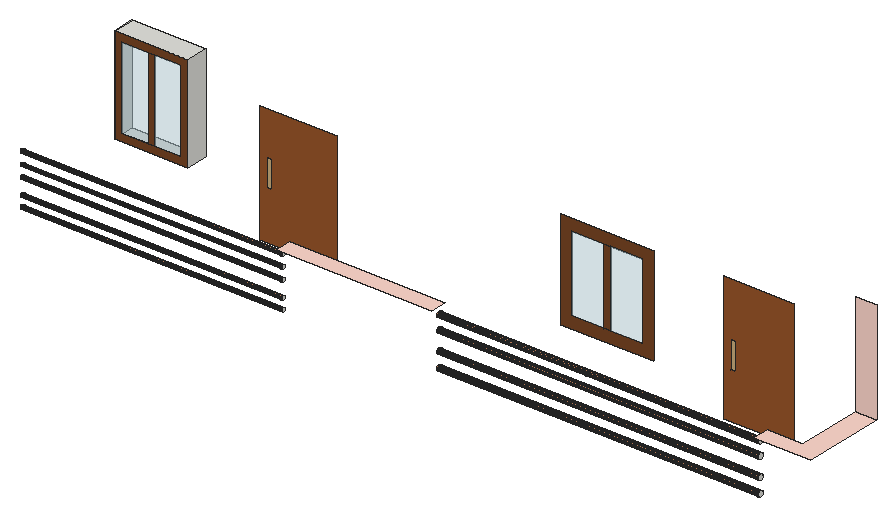
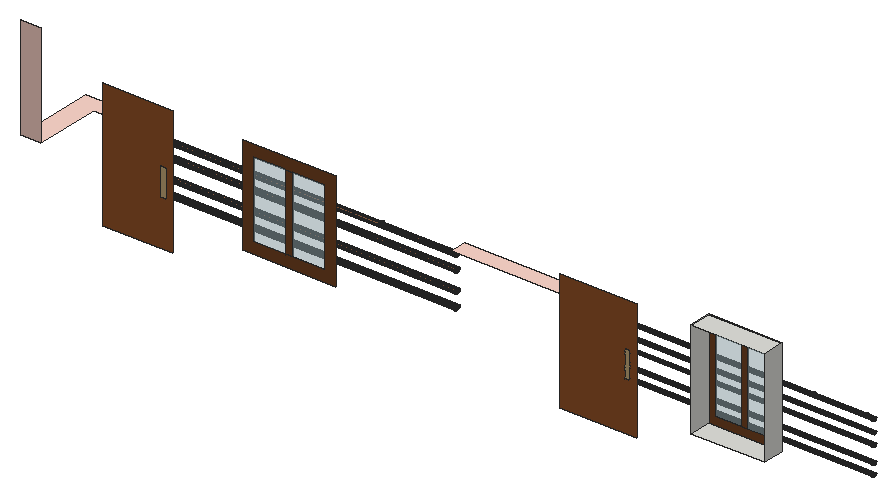
# SketchUp Ruby script. Lengths in inches.
U = 1.inch
M = Sketchup.active_model
def pt(a) = Geom::Point3d.new(a.map { |v| v * U })
def face(e, loops, mat)
  f = e.add_face(loops[0].map { |a| pt(a) })
  loops[1..].each { |l| e.add_face(l.map { |a| pt(a) }).erase! }
  f.material = f.back_material = mat if mat
  f
end
# faces: each face lists its corners as indices into pts; further lists are holes
def faces(e, pts, list, mat = nil) = list.each { |f| face(e, (f[0].is_a?(Array) ? f : [f]).map { |l| l.map { |i| pts[i] } }, mat) }
# xy, xz, yz: faces in a plane at the given z, y or x. An outline is a flat list of corners, or four numbers for a rectangle; further outlines are holes
def ring(l) = l.size == 4 ? [[l[0], l[1]], [l[2], l[1]], [l[2], l[3]], [l[0], l[3]]] : l.each_slice(2).to_a
def flat(e, list, mat, &to3) = list.each { |f| face(e, (f[0].is_a?(Array) ? f : [f]).map { |l| ring(l).map { |u, v| to3.(u, v) } }, mat) }
def xy(e, z, list, mat = nil) = flat(e, list, mat) { |x, y| [x, y, z] }
def xz(e, y, list, mat = nil) = flat(e, list, mat) { |x, z| [x, y, z] }
def yz(e, x, list, mat = nil) = flat(e, list, mat) { |y, z| [x, y, z] }
def lines(e, pts, list) = list.each { |a, b| e.add_line(pt(pts[a]), pt(pts[b])) }
# prism: a flat outline (further loops are holes) pulled along v
def prism(e, loops, v, mat = nil)
  f = face(e, loops, mat); d = Geom::Vector3d.new(v.map { |x| x * U })
  f.pushpull(f.normal.samedirection?(d) ? d.length : -d.length)
end
def box(e, o, s, mat = nil) = prism(e, [[o, [o[0] + s[0], o[1], o[2]], [o[0] + s[0], o[1] + s[1], o[2]], [o[0], o[1] + s[1], o[2]]]], [0, 0, s[2]], mat)
def at(x, y, z, deg = 0) = Geom::Transformation.translation(pt([x, y, z])) * Geom::Transformation.rotation(ORIGIN, Z_AXIS, deg.degrees)
def axes(o, x, y, z) = Geom::Transformation.new([*x, 0, *y, 0, *z, 0, *pt(o).to_a, 1])
def part(name) = M.definitions.add(name)
# library, detail: a bought-in or finely detailed component or shape, given as its bounding box
def library(name, o, s) = part(name).tap { |d| box(d.entities, o, s) }
def detail(e, o, s) = box(e.add_group.entities, o, s)
def put(e, d, t, mat = nil) = e.add_instance(d, t).tap { |i| i.material = mat if mat }
def group(e, t, mat = nil) = e.add_group.tap { |g| g.transformation = t; g.material = mat if mat }.entities
root = M.entities
M.materials.add("[Color B01]").color = [255, 216, 204]
M.materials.add("[Translucent Glass Safety]").color = [204, 235, 244]
M.materials["[Translucent Glass Safety]"].alpha = 0.5
M.materials.add("[Wood Cherry Original]").color = [152, 86, 42]
M.materials.add("[Wood Floor Light]").color = [204, 176, 127]
M.materials.add("[Wood Veneer 01]1").color = [120, 70, 37]
M.materials.add("[Wood Veneer 02]").color = [190, 128, 91]
xy(root,2135.23,[[206.78,571.9,480.91,653.97]])
xy(root,2168.9375,[[2479.625,285.86,2482.375,286.22,2484.9375,287.28,2487.14,288.97,2488.83,291.17,2489.89,293.73,2490.25,296.48,2489.89,299.23,2488.83,301.79,2487.14,303.99,2484.9375,305.68,2482.375,306.74,2479.625,307.11,2476.875,306.74,2474.3125,305.68,2472.11,303.99,2470.42,301.79,2469.36,299.23,2469,296.48,2469.36,293.73,2470.42,291.17,2472.11,288.97,2474.3125,287.28,2476.875,286.22]],"[Wood Veneer 02]")
xy(root,2169.25,[[530.58,291.11,532.59,291.37,534.45,292.15,536.06,293.38,537.29,294.98,538.07,296.85,538.33,298.86,538.07,300.86,537.29,302.73,536.06,304.34,534.45,305.57,532.59,306.34,530.58,306.61,528.57,306.34,526.7,305.57,525.1,304.34,523.87,302.73,523.09,300.86,522.83,298.86,523.09,296.85,523.87,294.98,525.1,293.38,526.7,292.15,528.57,291.37]])
xy(root,2169.6875,[[2192.5,285.86,2195.25,286.22,2197.8125,287.28,2200.01,288.97,2201.7,291.17,2202.76,293.73,2203.125,296.48,2202.76,299.23,2201.7,301.79,2200.01,303.99,2197.8125,305.68,2195.25,306.74,2192.5,307.11,2189.75,306.74,2187.1875,305.68,2184.99,303.99,2183.3,301.79,2182.24,299.23,2181.875,296.48,2182.24,293.73,2183.3,291.17,2184.99,288.97,2187.1875,287.28,2189.75,286.22]],"[Wood Veneer 02]")
xy(root,2170.12,[[988.02,291.11,990.02,291.37,991.89,292.15,993.5,293.38,994.73,294.98,994.75,295.02,981.29,295.02,981.31,294.98,982.54,293.38,984.14,292.15,986.01,291.37],[981.29,295.02,994.75,295.02,995.5,296.85,995.77,298.86,995.5,300.86,994.73,302.73,993.5,304.34,991.89,305.57,990.02,306.34,988.02,306.61,986.01,306.34,984.14,305.57,982.54,304.34,981.31,302.73,980.53,300.86,980.27,298.86,980.53,296.85]])
xy(root,2170.6875,[[748.77,291.11,750.77,291.37,752.64,292.15,754.25,293.38,755.48,294.98,756.25,296.85,756.52,298.86,756.25,300.86,755.48,302.73,754.25,304.34,752.64,305.57,750.77,306.34,748.77,306.61,746.76,306.34,744.89,305.57,743.29,304.34,742.06,302.73,741.28,300.86,741.02,298.86,741.28,296.85,742.06,294.98,743.29,293.38,744.89,292.15,746.76,291.37]])
xy(root,2171.4375,[[1711.75,285.86,1714.5,286.22,1717.0625,287.28,1719.26,288.97,1720.95,291.17,1722.01,293.73,1722.375,296.48,1722.01,299.23,1720.95,301.79,1719.26,303.99,1717.0625,305.68,1714.5,306.74,1711.75,307.11,1709,306.74,1706.4375,305.68,1704.24,303.99,1702.55,301.79,1701.49,299.23,1701.125,296.48,1701.49,293.73,1702.55,291.17,1704.24,288.97,1706.4375,287.28,1709,286.22]])
xy(root,2172.125,[[114.33,291.11,116.34,291.37,118.2,292.15,119.81,293.38,121.04,294.98,121.82,296.85,122.08,298.86,121.82,300.86,121.04,302.73,119.81,304.34,118.2,305.57,116.34,306.34,114.33,306.61,112.32,306.34,110.45,305.57,108.85,304.34,107.62,302.73,106.84,300.86,106.58,298.86,106.84,296.85,107.62,294.98,108.85,293.38,110.45,292.15,112.32,291.37]])
xy(root,2173.03,[[309.08,291.11,311.09,291.37,312.95,292.15,314.56,293.38,315.79,294.98,316.13,295.8,302.03,295.8,302.37,294.98,303.6,293.38,305.2,292.15,307.07,291.37],[302.03,295.8,316.13,295.8,316.57,296.85,316.83,298.86,316.57,300.86,315.79,302.73,314.56,304.34,312.95,305.57,312.23,305.87,305.93,305.87,305.2,305.57,303.6,304.34,302.37,302.73,301.59,300.86,301.33,298.86,301.59,296.85],[305.93,305.87,312.23,305.87,311.09,306.34,309.08,306.61,307.07,306.34]])
xy(root,2173.25,[[2741.25,285.86,2744,286.22,2746.5625,287.28,2748.76,288.97,2750.45,291.17,2751.51,293.73,2751.875,296.48,2751.51,299.23,2750.45,301.79,2748.76,303.99,2746.5625,305.68,2744,306.74,2741.25,307.11,2738.5,306.74,2735.9375,305.68,2733.74,303.99,2732.05,301.79,2730.99,299.23,2730.625,296.48,2730.99,293.73,2732.05,291.17,2733.74,288.97,2735.9375,287.28,2738.5,286.22]],"[Wood Veneer 02]")
xy(root,2176.5,[[1911.67,291.33,1930.2,291.33,1931.2,293.73,1931.5625,296.48,1931.2,299.23,1930.14,301.79,1928.45,303.99,1926.25,305.68,1923.6875,306.74,1921.5625,307.02,1920.3125,307.02,1918.1875,306.74,1915.625,305.68,1913.42,303.99,1911.74,301.79,1910.67,299.23,1910.3125,296.48,1910.67,293.73],[1920.3125,307.02,1921.5625,307.02,1920.9375,307.11]])
xy(root,2176.5,[[1920.9375,285.86,1923.6875,286.22,1926.25,287.28,1928.45,288.97,1930.14,291.17,1930.2,291.33,1911.67,291.33,1911.74,291.17,1913.42,288.97,1915.625,287.28,1918.1875,286.22]],"[Wood Veneer 02]")
xy(root,2195.8125,[[1053.15,267.5625,1631.4,328.8],[2829.41,267.5625,3040.15,267.5625,3040.15,571.9,2962.22,571.9,2962.22,328.8,2829.41,328.8]],"[Color B01]")
xy(root,2496.04,[[206.78,571.9,480.91,653.97]])
xz(root,571.9,[[2962.22,2195.8125,3040.15,2577.9375]],"[Color B01]")
xz(root,571.9,[[1909.23,2143.05,2027.6,2427.3],[2054.17,2143.05,2170.86,2427.3],[235.06,2163.5,333.67,2467.76],[357.21,2163.5,452.63,2467.76]],"[Translucent Glass Safety]")
xz(root,571.9,[[[747.7,1990.6,1033.12,2436.59],[772.37,2170.62,791.56,2274.62]],[[2473.97,2001.07,2732.77,2474.99],[2500.06,2170.62,2519.25,2274.62]]],"[Wood Cherry Original]")
xz(root,571.9,[[772.37,2170.62,791.56,2274.62],[2500.06,2170.62,2519.25,2274.62]],"[Wood Floor Light]")
xz(root,571.9,[[[1867.29,2101.11,2212.79,2469.24],[1909.23,2143.05,2170.86,2427.3]],[[206.78,2135.23,480.91,2496.04],[235.06,2163.5,452.63,2467.76]],[2027.6,2143.05,2054.17,2427.3],[333.67,2163.5,357.21,2467.76]],"[Wood Veneer 01]1")
yz(root,206.78,[[571.9,2135.23,653.97,2496.04]])
yz(root,480.91,[[571.9,2135.23,653.97,2496.04]])
yz(root,1053.15,[[300.84,1977.93,302.34,1978.13,303.74,1978.71,304.95,1979.63,305.87,1980.84,306.45,1982.24,306.65,1983.74,306.45,1985.25,305.87,1986.65,304.95,1987.85,303.74,1988.78,302.34,1989.36,300.84,1989.56,299.33,1989.36,297.93,1988.78,296.73,1987.85,295.8,1986.65,295.22,1985.25,295.02,1983.74,295.22,1982.24,295.8,1980.84,296.73,1979.63,297.93,1978.71,299.33,1978.13],[300.84,2017.49,302.34,2017.69,303.74,2018.27,304.95,2019.2,305.87,2020.4,306.45,2021.8,306.65,2023.31,306.45,2024.8125,305.87,2026.21,304.95,2027.42,303.74,2028.34,302.34,2028.92,300.84,2029.12,299.33,2028.92,297.93,2028.34,296.73,2027.42,295.8,2026.21,295.22,2024.8125,295.02,2023.31,295.22,2021.8,295.8,2020.4,296.73,2019.2,297.93,2018.27,299.33,2017.69],[300.84,2076.99,302.34,2077.19,303.74,2077.77,304.95,2078.7,305.87,2079.9,306.45,2081.3,306.65,2082.81,306.45,2084.3125,305.87,2085.71,304.95,2086.92,303.74,2087.84,302.34,2088.42,300.84,2088.62,299.33,2088.42,297.93,2087.84,296.73,2086.92,295.8,2085.71,295.22,2084.3125,295.02,2082.81,295.22,2081.3,295.8,2079.9,296.73,2078.7,297.93,2077.77,299.33,2077.19],[300.84,2119.12,302.34,2119.32,303.74,2119.9,304.95,2120.82,305.87,2122.03,306.45,2123.43,306.65,2124.93,306.45,2126.4375,305.87,2127.84,304.95,2129.04,303.74,2129.97,302.34,2130.55,300.84,2130.74,299.33,2130.55,297.93,2129.97,296.73,2129.04,295.8,2127.84,295.22,2126.4375,295.02,2124.93,295.22,2123.43,295.8,2122.03,296.73,2120.82,297.93,2119.9,299.33,2119.32],[300.84,2164.31,302.34,2164.51,303.74,2165.09,304.95,2166.01,305.87,2167.21,306.45,2168.62,306.65,2170.12,306.45,2171.625,305.87,2173.03,304.95,2174.23,303.74,2175.15,302.34,2175.73,300.84,2175.93,299.33,2175.73,297.93,2175.15,296.73,2174.23,295.8,2173.03,295.22,2171.625,295.02,2170.12,295.22,2168.62,295.8,2167.21,296.73,2166.01,297.93,2165.09,299.33,2164.51]])
yz(root,2829.41,[[299.17,1985.65,301.52,1985.96,303.71,1986.87,305.58,1988.31,307.02,1990.18,307.93,1992.37,308.24,1994.72,307.93,1997.0625,307.02,1999.25,305.58,2001.125,303.71,2002.5625,301.52,2003.47,299.17,2003.78,296.83,2003.47,294.64,2002.5625,292.77,2001.125,291.33,1999.25,290.42,1997.0625,290.11,1994.72,290.42,1992.37,291.33,1990.18,292.77,1988.31,294.64,1986.87,296.83,1985.96],[299.17,2040.72,301.52,2041.02,303.71,2041.93,305.58,2043.37,307.02,2045.25,307.93,2047.43,308.24,2049.78,307.93,2052.125,307.02,2054.31,305.58,2056.1875,303.71,2057.625,301.52,2058.53,299.17,2058.84,296.83,2058.53,294.64,2057.625,292.77,2056.1875,291.33,2054.31,290.42,2052.125,290.11,2049.78,290.42,2047.43,291.33,2045.25,292.77,2043.37,294.64,2041.93,296.83,2041.02],[299.17,2111.15,301.52,2111.46,303.71,2112.37,305.58,2113.81,307.02,2115.68,307.93,2117.87,308.24,2120.22,307.93,2122.5625,307.02,2124.75,305.58,2126.625,303.71,2128.0625,301.52,2128.97,299.17,2129.28,296.83,2128.97,294.64,2128.0625,292.77,2126.625,291.33,2124.75,290.42,2122.5625,290.11,2120.22,290.42,2117.87,291.33,2115.68,292.77,2113.81,294.64,2112.37,296.83,2111.46],[299.17,2162.9,301.52,2163.21,303.71,2164.12,305.58,2165.56,307.02,2167.43,307.93,2169.62,308.24,2171.97,307.93,2174.3125,307.02,2176.5,305.58,2178.375,303.71,2179.8125,301.52,2180.72,299.17,2181.03,296.83,2180.72,294.64,2179.8125,292.77,2178.375,291.33,2176.5,290.42,2174.3125,290.11,2171.97,290.42,2169.62,291.33,2167.43,292.77,2165.56,294.64,2164.12,296.83,2163.21]])
p = [[1053.15,300.84,1977.93],[1053.15,299.33,1978.13],[77.93,299.33,1978.13],[77.93,300.84,1977.93],[1053.15,302.34,1978.13],[77.93,302.34,1978.13],
  [1053.15,297.93,1978.71],[77.93,297.93,1978.71],[1053.15,303.74,1978.71],[77.93,303.74,1978.71],[1053.15,296.73,1979.63],[77.93,296.73,1979.63],
  [1053.15,304.95,1979.63],[77.93,304.95,1979.63],[1053.15,295.8,1980.84],[77.93,295.8,1980.84],[1053.15,305.87,1980.84],[77.93,305.87,1980.84],
  [1053.15,295.22,1982.24],[77.93,295.22,1982.24],[1053.15,306.45,1982.24],[77.93,306.45,1982.24],[1053.15,295.02,1983.74],[77.93,295.02,1983.74],
  [1053.15,306.65,1983.74],[77.93,306.65,1983.74],[1053.15,295.22,1985.25],[77.93,295.22,1985.25],[1053.15,306.45,1985.25],[77.93,306.45,1985.25],
  [1053.15,295.8,1986.65],[77.93,295.8,1986.65],[1053.15,305.87,1986.65],[77.93,305.87,1986.65],[2829.41,299.17,1985.65],[2829.41,296.83,1985.96],
  [1631.4,296.83,1985.96],[1631.4,299.17,1985.65],[2829.41,301.52,1985.96],[1631.4,301.52,1985.96],[2829.41,294.64,1986.87],[1631.4,294.64,1986.87],
  [2829.41,303.71,1986.87],[1631.4,303.71,1986.87],[1053.15,296.73,1987.85],[77.93,296.73,1987.85],[1053.15,304.95,1987.85],[77.93,304.95,1987.85],
  [2829.41,292.77,1988.31],[1631.4,292.77,1988.31],[2829.41,305.58,1988.31],[1631.4,305.58,1988.31],[1053.15,297.93,1988.78],[77.93,297.93,1988.78],
  [1053.15,303.74,1988.78],[77.93,303.74,1988.78],[2829.41,291.33,1990.18],[1631.4,291.33,1990.18],[2829.41,307.02,1990.18],[1631.4,307.02,1990.18],
  [1053.15,299.33,1989.36],[77.93,299.33,1989.36],[1053.15,302.34,1989.36],[77.93,302.34,1989.36],[1053.15,300.84,1989.56],[77.93,300.84,1989.56],
  [2829.41,290.42,1992.37],[1631.4,290.42,1992.37],[2829.41,307.93,1992.37],[1631.4,307.93,1992.37],[2829.41,290.11,1994.72],[1631.4,290.11,1994.72],
  [2829.41,308.24,1994.72],[1631.4,308.24,1994.72],[2829.41,290.42,1997.0625],[1631.4,290.42,1997.0625],[2829.41,307.93,1997.0625],[1631.4,307.93,1997.0625],
  [2829.41,291.33,1999.25],[1631.4,291.33,1999.25],[2829.41,307.02,1999.25],[1631.4,307.02,1999.25],[2829.41,292.77,2001.125],[1631.4,292.77,2001.125],
  [2829.41,305.58,2001.125],[1631.4,305.58,2001.125],[2829.41,294.64,2002.5625],[1631.4,294.64,2002.5625],[2829.41,303.71,2002.5625],[1631.4,303.71,2002.5625],
  [2829.41,296.83,2003.47],[1631.4,296.83,2003.47],[2829.41,301.52,2003.47],[1631.4,301.52,2003.47],[2829.41,299.17,2003.78],[1631.4,299.17,2003.78],
  [1053.15,300.84,2017.49],[1053.15,299.33,2017.69],[77.93,299.33,2017.69],[77.93,300.84,2017.49],[1053.15,302.34,2017.69],[77.93,302.34,2017.69],
  [1053.15,297.93,2018.27],[77.93,297.93,2018.27],[1053.15,303.74,2018.27],[77.93,303.74,2018.27],[1053.15,296.73,2019.2],[77.93,296.73,2019.2],
  [1053.15,304.95,2019.2],[77.93,304.95,2019.2],[1053.15,295.8,2020.4],[77.93,295.8,2020.4],[1053.15,305.87,2020.4],[77.93,305.87,2020.4],
  [1053.15,295.22,2021.8],[77.93,295.22,2021.8],[1053.15,306.45,2021.8],[77.93,306.45,2021.8],[1053.15,295.02,2023.31],[77.93,295.02,2023.31],
  [1053.15,306.65,2023.31],[77.93,306.65,2023.31],[1053.15,295.22,2024.8125],[77.93,295.22,2024.8125],[1053.15,306.45,2024.8125],[77.93,306.45,2024.8125],
  [1053.15,295.8,2026.21],[77.93,295.8,2026.21],[1053.15,305.87,2026.21],[77.93,305.87,2026.21],[1053.15,296.73,2027.42],[77.93,296.73,2027.42],
  [1053.15,304.95,2027.42],[77.93,304.95,2027.42],[1053.15,297.93,2028.34],[77.93,297.93,2028.34],[1053.15,303.74,2028.34],[77.93,303.74,2028.34],
  [1053.15,299.33,2028.92],[77.93,299.33,2028.92],[1053.15,302.34,2028.92],[77.93,302.34,2028.92],[1053.15,300.84,2029.12],[77.93,300.84,2029.12],
  [2829.41,299.17,2040.72],[2829.41,296.83,2041.02],[1631.4,296.83,2041.02],[1631.4,299.17,2040.72],[2829.41,301.52,2041.02],[1631.4,301.52,2041.02],
  [2829.41,294.64,2041.93],[1631.4,294.64,2041.93],[2829.41,303.71,2041.93],[1631.4,303.71,2041.93],[2829.41,292.77,2043.37],[1631.4,292.77,2043.37],
  [2829.41,305.58,2043.37],[1631.4,305.58,2043.37],[2829.41,291.33,2045.25],[1631.4,291.33,2045.25],[2829.41,307.02,2045.25],[1631.4,307.02,2045.25],
  [2829.41,290.42,2047.43],[1631.4,290.42,2047.43],[2829.41,307.93,2047.43],[1631.4,307.93,2047.43],[2829.41,290.11,2049.78],[1631.4,290.11,2049.78],
  [2829.41,308.24,2049.78],[1631.4,308.24,2049.78],[2829.41,290.42,2052.125],[1631.4,290.42,2052.125],[2829.41,307.93,2052.125],[1631.4,307.93,2052.125],
  [2829.41,291.33,2054.31],[1631.4,291.33,2054.31],[2829.41,307.02,2054.31],[1631.4,307.02,2054.31],[2829.41,292.77,2056.1875],[1631.4,292.77,2056.1875],
  [2829.41,305.58,2056.1875],[1631.4,305.58,2056.1875],[2829.41,294.64,2057.625],[1631.4,294.64,2057.625],[2829.41,303.71,2057.625],[1631.4,303.71,2057.625],
  [2829.41,296.83,2058.53],[1631.4,296.83,2058.53],[2829.41,301.52,2058.53],[1631.4,301.52,2058.53],[2829.41,299.17,2058.84],[1631.4,299.17,2058.84],
  [1053.15,300.84,2076.99],[1053.15,299.33,2077.19],[77.93,299.33,2077.19],[77.93,300.84,2076.99],[1053.15,302.34,2077.19],[77.93,302.34,2077.19],
  [1053.15,297.93,2077.77],[77.93,297.93,2077.77],[1053.15,303.74,2077.77],[77.93,303.74,2077.77],[1053.15,296.73,2078.7],[77.93,296.73,2078.7],
  [1053.15,304.95,2078.7],[77.93,304.95,2078.7],[1053.15,295.8,2079.9],[77.93,295.8,2079.9],[1053.15,305.87,2079.9],[77.93,305.87,2079.9],
  [1053.15,295.22,2081.3],[77.93,295.22,2081.3],[1053.15,306.45,2081.3],[77.93,306.45,2081.3],[1053.15,295.02,2082.81],[77.93,295.02,2082.81],
  [1053.15,306.65,2082.81],[77.93,306.65,2082.81],[1053.15,295.22,2084.3125],[77.93,295.22,2084.3125],[1053.15,306.45,2084.3125],[77.93,306.45,2084.3125],
  [1053.15,295.8,2085.71],[77.93,295.8,2085.71],[1053.15,305.87,2085.71],[77.93,305.87,2085.71],[1053.15,296.73,2086.92],[77.93,296.73,2086.92],
  [1053.15,304.95,2086.92],[77.93,304.95,2086.92],[1053.15,297.93,2087.84],[77.93,297.93,2087.84],[1053.15,303.74,2087.84],[77.93,303.74,2087.84],
  [1053.15,299.33,2088.42],[77.93,299.33,2088.42],[1053.15,302.34,2088.42],[77.93,302.34,2088.42],[1053.15,300.84,2088.62],[77.93,300.84,2088.62],
  [2829.41,299.17,2111.15],[2829.41,296.83,2111.46],[1631.4,296.83,2111.46],[1631.4,299.17,2111.15],[2829.41,301.52,2111.46],[1631.4,301.52,2111.46],
  [2829.41,294.64,2112.37],[1631.4,294.64,2112.37],[2829.41,303.71,2112.37],[1631.4,303.71,2112.37],[2829.41,292.77,2113.81],[1631.4,292.77,2113.81],
  [2829.41,305.58,2113.81],[1631.4,305.58,2113.81],[2829.41,291.33,2115.68],[1631.4,291.33,2115.68],[2829.41,307.02,2115.68],[1631.4,307.02,2115.68],
  [2829.41,290.42,2117.87],[1631.4,290.42,2117.87],[2829.41,307.93,2117.87],[1631.4,307.93,2117.87],[2829.41,290.11,2120.22],[1631.4,290.11,2120.22],
  [2829.41,308.24,2120.22],[1631.4,308.24,2120.22],[1053.15,300.84,2119.12],[1053.15,299.33,2119.32],[77.93,299.33,2119.32],[77.93,300.84,2119.12],
  [1053.15,302.34,2119.32],[77.93,302.34,2119.32],[1053.15,297.93,2119.9],[77.93,297.93,2119.9],[1053.15,303.74,2119.9],[77.93,303.74,2119.9],
  [1053.15,296.73,2120.82],[77.93,296.73,2120.82],[1053.15,304.95,2120.82],[77.93,304.95,2120.82],[2829.41,290.42,2122.5625],[1631.4,290.42,2122.5625],
  [2829.41,307.93,2122.5625],[1631.4,307.93,2122.5625],[1053.15,295.8,2122.03],[77.93,295.8,2122.03],[1053.15,305.87,2122.03],[77.93,305.87,2122.03],
  [1053.15,295.22,2123.43],[77.93,295.22,2123.43],[1053.15,306.45,2123.43],[77.93,306.45,2123.43],[2829.41,291.33,2124.75],[1631.4,291.33,2124.75],
  [2829.41,307.02,2124.75],[1631.4,307.02,2124.75],[1053.15,295.02,2124.93],[77.93,295.02,2124.93],[1053.15,306.65,2124.93],[77.93,306.65,2124.93],
  [2829.41,292.77,2126.625],[1631.4,292.77,2126.625],[2829.41,305.58,2126.625],[1631.4,305.58,2126.625],[1053.15,295.22,2126.4375],[77.93,295.22,2126.4375],
  [1053.15,306.45,2126.4375],[77.93,306.45,2126.4375],[1053.15,295.8,2127.84],[77.93,295.8,2127.84],[1053.15,305.87,2127.84],[77.93,305.87,2127.84],
  [2829.41,294.64,2128.0625],[1631.4,294.64,2128.0625],[2829.41,303.71,2128.0625],[1631.4,303.71,2128.0625],[1053.15,296.73,2129.04],[77.93,296.73,2129.04],
  [1053.15,304.95,2129.04],[77.93,304.95,2129.04],[2829.41,296.83,2128.97],[1631.4,296.83,2128.97],[2829.41,301.52,2128.97],[1631.4,301.52,2128.97],
  [1053.15,297.93,2129.97],[77.93,297.93,2129.97],[2829.41,299.17,2129.28],[1631.4,299.17,2129.28],[1053.15,303.74,2129.97],[77.93,303.74,2129.97],
  [1053.15,299.33,2130.55],[77.93,299.33,2130.55],[1053.15,302.34,2130.55],[77.93,302.34,2130.55],[1053.15,300.84,2130.74],[77.93,300.84,2130.74],
  [2829.41,299.17,2162.9],[2829.41,296.83,2163.21],[1631.4,296.83,2163.21],[1631.4,299.17,2162.9],[2829.41,301.52,2163.21],[1631.4,301.52,2163.21],
  [2829.41,294.64,2164.12],[1631.4,294.64,2164.12],[2829.41,303.71,2164.12],[1631.4,303.71,2164.12],[2829.41,292.77,2165.56],[1631.4,292.77,2165.56],
  [2829.41,305.58,2165.56],[1631.4,305.58,2165.56],[1053.15,300.84,2164.31],[1053.15,299.33,2164.51],[77.93,299.33,2164.51],[77.93,300.84,2164.31],
  [1053.15,302.34,2164.51],[77.93,302.34,2164.51],[1053.15,297.93,2165.09],[77.93,297.93,2165.09],[1053.15,303.74,2165.09],[77.93,303.74,2165.09],
  [1053.15,296.73,2166.01],[77.93,296.73,2166.01],[1053.15,304.95,2166.01],[77.93,304.95,2166.01],[2829.41,291.33,2167.43],[1631.4,291.33,2167.43],
  [2829.41,307.02,2167.43],[1631.4,307.02,2167.43],[1053.15,295.8,2167.21],[77.93,295.8,2167.21],[1053.15,305.87,2167.21],[77.93,305.87,2167.21],
  [1053.15,295.22,2168.62],[77.93,295.22,2168.62],[1053.15,306.45,2168.62],[77.93,306.45,2168.62],[2829.41,290.42,2169.62],[1631.4,290.42,2169.62],
  [2829.41,307.93,2169.62],[1631.4,307.93,2169.62],[1053.15,295.02,2170.12],[994.75,295.02,2170.12],[981.29,295.02,2170.12],[77.93,295.02,2170.12],
  [1053.15,306.65,2170.12],[77.93,306.65,2170.12],[2829.41,290.11,2171.97],[1631.4,290.11,2171.97],[2829.41,308.24,2171.97],[1631.4,308.24,2171.97],
  [1053.15,295.22,2171.625],[77.93,295.22,2171.625],[1053.15,306.45,2171.625],[77.93,306.45,2171.625],[1053.15,295.8,2173.03],[316.13,295.8,2173.03],
  [302.03,295.8,2173.03],[77.93,295.8,2173.03],[1053.15,305.87,2173.03],[77.93,305.87,2173.03],[305.93,305.87,2173.03],[312.23,305.87,2173.03],
  [2829.41,290.42,2174.3125],[1631.4,290.42,2174.3125],[2829.41,307.93,2174.3125],[1631.4,307.93,2174.3125],[1053.15,296.73,2174.23],[77.93,296.73,2174.23],
  [1053.15,304.95,2174.23],[77.93,304.95,2174.23],[1053.15,297.93,2175.15],[77.93,297.93,2175.15],[1053.15,303.74,2175.15],[77.93,303.74,2175.15],
  [2829.41,291.33,2176.5],[1930.2,291.33,2176.5],[1911.67,291.33,2176.5],[1631.4,291.33,2176.5],[2829.41,307.02,2176.5],[1631.4,307.02,2176.5],
  [1920.3125,307.02,2176.5],[1921.5625,307.02,2176.5],[1053.15,299.33,2175.73],[77.93,299.33,2175.73],[1053.15,302.34,2175.73],[77.93,302.34,2175.73],
  [1053.15,300.84,2175.93],[77.93,300.84,2175.93],[2829.41,292.77,2178.375],[1631.4,292.77,2178.375],[2829.41,305.58,2178.375],[1631.4,305.58,2178.375],
  [2829.41,294.64,2179.8125],[1631.4,294.64,2179.8125],[2829.41,303.71,2179.8125],[1631.4,303.71,2179.8125],[2829.41,296.83,2180.72],[1631.4,296.83,2180.72],
  [2829.41,301.52,2180.72],[1631.4,301.52,2180.72],[2829.41,299.17,2181.03],[1631.4,299.17,2181.03]]
faces(root,p,[[0,1,2,3],[4,0,3,5],[1,6,7,2],[8,4,5,9],[6,10,11,7],[12,8,9,13],[10,14,15,11],[16,12,13,17],
  [14,18,19,15],[20,16,17,21],[18,22,23,19],[24,20,21,25],[22,26,27,23],[28,24,25,29],[26,30,31,27],[32,28,29,33],
  [34,35,36,37],[38,34,37,39],[35,40,41,36],[42,38,39,43],[30,44,45,31],[46,32,33,47],[40,48,49,41],[50,42,43,51],
  [44,52,53,45],[54,46,47,55],[48,56,57,49],[58,50,51,59],[52,60,61,53],[62,54,55,63],[60,64,65,61],[64,62,63,65],
  [56,66,67,57],[68,58,59,69],[66,70,71,67],[72,68,69,73],[70,74,75,71],[76,72,73,77],[74,78,79,75],[80,76,77,81],
  [78,82,83,79],[84,80,81,85],[82,86,87,83],[88,84,85,89],[86,90,91,87],[92,88,89,93],[90,94,95,91],[94,92,93,95],
  [96,97,98,99],[100,96,99,101],[97,102,103,98],[104,100,101,105],[102,106,107,103],[108,104,105,109],[106,110,111,107],[112,108,109,113],
  [110,114,115,111],[116,112,113,117],[114,118,119,115],[120,116,117,121],[118,122,123,119],[124,120,121,125],[122,126,127,123],[128,124,125,129],
  [126,130,131,127],[132,128,129,133],[130,134,135,131],[136,132,133,137],[134,138,139,135],[140,136,137,141],[138,142,143,139],[142,140,141,143],
  [144,145,146,147],[148,144,147,149],[145,150,151,146],[152,148,149,153],[150,154,155,151],[156,152,153,157],[154,158,159,155],[160,156,157,161],
  [158,162,163,159],[164,160,161,165],[162,166,167,163],[168,164,165,169],[166,170,171,167],[172,168,169,173],[170,174,175,171],[176,172,173,177],
  [174,178,179,175],[180,176,177,181],[178,182,183,179],[184,180,181,185],[182,186,187,183],[188,184,185,189],[186,190,191,187],[190,188,189,191],
  [192,193,194,195],[196,192,195,197],[193,198,199,194],[200,196,197,201],[198,202,203,199],[204,200,201,205],[202,206,207,203],[208,204,205,209],
  [206,210,211,207],[212,208,209,213],[210,214,215,211],[216,212,213,217],[214,218,219,215],[220,216,217,221],[218,222,223,219],[224,220,221,225],
  [222,226,227,223],[228,224,225,229],[226,230,231,227],[232,228,229,233],[230,234,235,231],[236,232,233,237],[234,238,239,235],[238,236,237,239],
  [240,241,242,243],[244,240,243,245],[241,246,247,242],[248,244,245,249],[246,250,251,247],[252,248,249,253],[250,254,255,251],[256,252,253,257],
  [254,258,259,255],[260,256,257,261],[258,262,263,259],[264,260,261,265],[266,267,268,269],[270,266,269,271],[267,272,273,268],[274,270,271,275],
  [272,276,277,273],[278,274,275,279],[262,280,281,263],[282,264,265,283],[276,284,285,277],[286,278,279,287],[284,288,289,285],[290,286,287,291],
  [280,292,293,281],[294,282,283,295],[288,296,297,289],[298,290,291,299],[292,300,301,293],[302,294,295,303],[296,304,305,297],[306,298,299,307],
  [304,308,309,305],[310,306,307,311],[300,312,313,301],[314,302,303,315],[308,316,317,309],[318,310,311,319],[312,320,321,313],[322,314,315,323],
  [316,324,325,317],[320,326,327,321],[326,322,323,327],[328,318,319,329],[324,330,331,325],[332,328,329,333],[330,334,335,331],[334,332,333,335],
  [336,337,338,339],[340,336,339,341],[337,342,343,338],[344,340,341,345],[342,346,347,343],[348,344,345,349],[350,351,352,353],[354,350,353,355],
  [351,356,357,352],[358,354,355,359],[356,360,361,357],[362,358,359,363],[346,364,365,347],[366,348,349,367],[360,368,369,361],[370,362,363,371],
  [368,372,373,369],[374,370,371,375],[364,376,377,365],[378,366,367,379],[372,380,381,382,383,373],[384,374,375,385],[376,386,387,377],[388,378,379,389],
  [380,390,391,383,382,381],[392,384,385,393],[390,394,395,396,397,391],[398,392,393,399,400,401],[386,402,403,387],[404,388,389,405],[394,406,407,397,396,395],[408,398,401,400,399,409],
  [406,410,411,407],[412,408,409,413],[402,414,415,416,417,403],[418,404,405,419,420,421],[410,422,423,411],[424,412,413,425],[422,426,427,423],[426,424,425,427],
  [414,428,429,417,416,415],[430,418,421,420,419,431],[428,432,433,429],[434,430,431,435],[432,436,437,433],[438,434,435,439],[436,440,441,437],[440,438,439,441]],"[Wood Veneer 02]")
